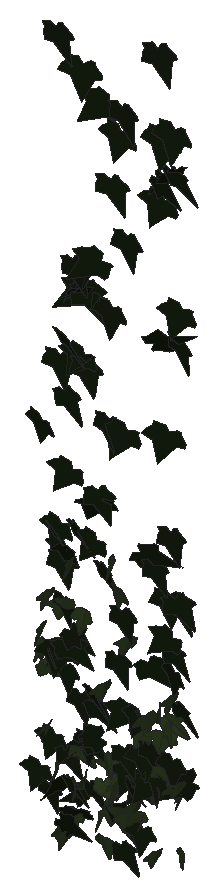
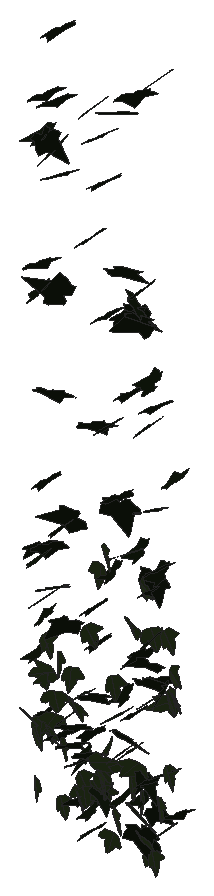
# SketchUp Ruby script. Lengths in inches.
U = 1.inch
M = Sketchup.active_model
def pt(a) = Geom::Point3d.new(a.map { |v| v * U })
def face(e, loops, mat)
  f = e.add_face(loops[0].map { |a| pt(a) })
  loops[1..].each { |l| e.add_face(l.map { |a| pt(a) }).erase! }
  f.material = f.back_material = mat if mat
  f
end
# faces: each face lists its corners as indices into pts; further lists are holes
def faces(e, pts, list, mat = nil) = list.each { |f| face(e, (f[0].is_a?(Array) ? f : [f]).map { |l| l.map { |i| pts[i] } }, mat) }
# xy, xz, yz: faces in a plane at the given z, y or x. An outline is a flat list of corners, or four numbers for a rectangle; further outlines are holes
def ring(l) = l.size == 4 ? [[l[0], l[1]], [l[2], l[1]], [l[2], l[3]], [l[0], l[3]]] : l.each_slice(2).to_a
def flat(e, list, mat, &to3) = list.each { |f| face(e, (f[0].is_a?(Array) ? f : [f]).map { |l| ring(l).map { |u, v| to3.(u, v) } }, mat) }
def xy(e, z, list, mat = nil) = flat(e, list, mat) { |x, y| [x, y, z] }
def xz(e, y, list, mat = nil) = flat(e, list, mat) { |x, z| [x, y, z] }
def yz(e, x, list, mat = nil) = flat(e, list, mat) { |y, z| [x, y, z] }
def lines(e, pts, list) = list.each { |a, b| e.add_line(pt(pts[a]), pt(pts[b])) }
# prism: a flat outline (further loops are holes) pulled along v
def prism(e, loops, v, mat = nil)
  f = face(e, loops, mat); d = Geom::Vector3d.new(v.map { |x| x * U })
  f.pushpull(f.normal.samedirection?(d) ? d.length : -d.length)
end
def box(e, o, s, mat = nil) = prism(e, [[o, [o[0] + s[0], o[1], o[2]], [o[0] + s[0], o[1] + s[1], o[2]], [o[0], o[1] + s[1], o[2]]]], [0, 0, s[2]], mat)
def at(x, y, z, deg = 0) = Geom::Transformation.translation(pt([x, y, z])) * Geom::Transformation.rotation(ORIGIN, Z_AXIS, deg.degrees)
def axes(o, x, y, z) = Geom::Transformation.new([*x, 0, *y, 0, *z, 0, *pt(o).to_a, 1])
def part(name) = M.definitions.add(name)
# library, detail: a bought-in or finely detailed component or shape, given as its bounding box
def library(name, o, s) = part(name).tap { |d| box(d.entities, o, s) }
def detail(e, o, s) = box(e.add_group.entities, o, s)
def put(e, d, t, mat = nil) = e.add_instance(d, t).tap { |i| i.material = mat if mat }
def group(e, t, mat = nil) = e.add_group.tap { |g| g.transformation = t; g.material = mat if mat }.entities
root = M.entities
M.materials.add("1026 AP 7946 SUNNY SIDE UP").color = [254, 231, 186]
M.materials.add("efeu1").color = [18, 25, 13]
M.materials.add("efeu2").color = [43, 57, 29]
c1 = part("ivyleaf_9")
p = [[1.54,2.16,1.25],[1.36,2.04,1.19],[-0.21,0.99,0.68],[-0.71,1.11,0.82],[-0.85,0.86,0.67],[-0.8,0.17,0.21],
  [-0.9,-0.01,0.1],[-0.67,-0.16,-0.02],[-0.08,-0.08,-0.05],[-0.03,-0.6,-0.4],[0.65,-0.88,-0.66],[0.83,-0.6,-0.49],
  [1.29,-0.42,-0.43],[1.8125,-0.07,-0.26],[1.21,0.44,0.15]]
faces(c1.entities,p,[[0,1,2,3,4,5,6,7,8,9,10,11,12,13,14]],"efeu1")
c2 = part("ivyleaf_10")
p = [[0,0.5,-0.03],[-0.0625,2.02,-0.43],[-0.19,2.01,-0.46],[-0.54,1.05,-0.29],[-0.52,0.625,-0.18],[-0.83,0.76,-0.28],
  [-1.16,0.64,-0.33],[-1.15,0.33,-0.24],[-0.77,-0.39,0.02],[-0.3,-0.51,0.16],[0.04,-0.48,0.23],[-0.02,2.01,-0.4375],
  [-0.06,2.01,-0.43],[0.04,-0.49,0.23],[0.67,-0.49,0.14],[1.38,0.36,-0.2],[1.375,0.51,-0.24],[0.81,0.65,-0.19],
  [0.62,0.59,-0.15],[0.6,1.09,-0.28],[0.5,1.23,-0.31]]
faces(c2.entities,p,[[0,1,2,3,4,5,6,7,8,9,10],[11,12,0,13,14,15,16,17,18,19,20]],"efeu2")
put(root,c1,axes([126.55,212.5,293.42],[-0.23595,-0.32373,0.07815],[-0.0196,-0.0797,-0.36738],[0.52312,-0.149,0.02148]),"1026 AP 7946 SUNNY SIDE UP")
put(root,c2,axes([126.6,212.58,298.9375],[0.33541,-0.32342,0.04435],[0.00742,-0.05056,-0.39867],[0.51336,0.21204,-0.02322]),"1026 AP 7946 SUNNY SIDE UP")
put(root,c1,axes([126.43,212.75,308.94],[-0.07996,-0.33132,0.24837],[0.06056,-0.24759,-0.34096],[0.6432,-0.01787,0.06298]),"1026 AP 7946 SUNNY SIDE UP")
put(root,c2,axes([126.68,212.49,299.83],[0.19146,-0.33124,0.17534],[0.08492,-0.16347,-0.36448],[0.58076,0.1331,-0.00451]),"1026 AP 7946 SUNNY SIDE UP")
put(root,c2,axes([126.76,212.63,298.82],[0.18874,-0.3655,0.00071],[-0.00202,-0.00333,-0.39634],[0.57473,0.12002,-0.00162]),"1026 AP 7946 SUNNY SIDE UP")
put(root,c2,axes([126.86,212.58,295.33],[0.04072,-0.37809,-0.0197],[-0.00933,0.01661,-0.39029],[0.59504,0.02613,-0.00477]),"1026 AP 7946 SUNNY SIDE UP")
put(root,c2,axes([127.04,212.45,301.48],[-0.00893,-0.38837,0.07664],[0.00467,-0.07665,-0.40057],[0.62242,-0.005,0.00411]),"1026 AP 7946 SUNNY SIDE UP")
put(root,c1,axes([126.87,212.68,292.64],[0.09245,-0.36281,0.01679],[0.01263,-0.01729,-0.37871],[0.57108,0.05912,0.00566]),"1026 AP 7946 SUNNY SIDE UP")
put(root,c1,axes([127.21,212.57,295.04],[-0.22827,-0.32169,0.12073],[0.01396,-0.13272,-0.35918],[0.53916,-0.13276,0.06041]),"1026 AP 7946 SUNNY SIDE UP")
put(root,c1,axes([127.27,212.25,299.08],[0.34526,-0.127,-0.30141],[-0.36637,0.17741,-0.25908],[0.34095,0.31924,0.02682]),"1026 AP 7946 SUNNY SIDE UP")
put(root,c2,axes([127.05,212.27,298.3125],[-0.29857,-0.12669,-0.31996],[0.46627,0.10165,-0.22943],[0.24425,-0.34891,0.04685]),"1026 AP 7946 SUNNY SIDE UP")
put(root,c2,axes([127.45,212.39,293.61],[0.10401,-0.31533,-0.20418],[-0.06261,0.19233,-0.33079],[0.58077,0.07721,0.00091]),"1026 AP 7946 SUNNY SIDE UP")
put(root,c1,axes([127.35,212.77,304.55],[-0.20686,-0.34979,0.14767],[-0.03951,-0.14544,-0.38493],[0.59429,-0.13143,0.02581]),"1026 AP 7946 SUNNY SIDE UP")
put(root,c1,axes([127.13,212.6,304.4],[0.4088,-0.31305,0.04436],[0.01422,-0.05066,-0.41871],[0.49707,0.25891,-0.0245]),"1026 AP 7946 SUNNY SIDE UP")
put(root,c1,axes([127.34,212.79,312.13],[-0.07721,-0.4209,-0.01707],[0.03892,0.01137,-0.43582],[0.66105,-0.04983,0.02367]),"1026 AP 7946 SUNNY SIDE UP")
put(root,c1,axes([127.73,212.45,293.22],[-0.14938,0.12869,-0.33624],[0.15491,-0.31553,-0.15919],[-0.53058,-0.12835,0.04819]),"1026 AP 7946 SUNNY SIDE UP")
put(root,c2,axes([127.68,212.5,291.06],[-0.0168,-0.36717,-0.02915],[0.02359,0.02577,-0.37798],[0.57833,-0.01172,0.01457]),"1026 AP 7946 SUNNY SIDE UP")
put(root,c1,axes([127.8,212.3,303.91],[0.42656,0.03098,-0.31665],[-0.45801,-0.11133,-0.27689],[-0.16267,0.3947,-0.05074]),"1026 AP 7946 SUNNY SIDE UP")
put(root,c1,axes([127.62,212.32,299.22],[-0.33432,-0.31974,-0.07946],[0.07534,0.05857,-0.39516],[0.511,-0.21783,0.00627]),"1026 AP 7946 SUNNY SIDE UP")
put(root,c1,axes([127.39,212.52,327.11],[0.15416,-0.46374,-0.03363],[0.00581,0.03145,-0.48801],[0.73069,0.09759,0.01097]),"1026 AP 7946 SUNNY SIDE UP")
put(root,c2,axes([127.81,212.42,301.33],[-0.34287,-0.31244,0.0685],[-0.01836,-0.0748,-0.3915],[0.50254,-0.2159,0.03244]),"1026 AP 7946 SUNNY SIDE UP")
put(root,c1,axes([127.97,212.71,299.18],[-0.54854,-0.15041,0.05138],[-0.05926,-0.04051,-0.39094],[0.24246,-0.35019,0.0207]),"1026 AP 7946 SUNNY SIDE UP")
put(root,c1,axes([127.82,212.875,307.15],[-0.38359,-0.29355,0.15153],[-0.00447,-0.18329,-0.37848],[0.51744,-0.21919,0.10907]),"1026 AP 7946 SUNNY SIDE UP")
put(root,c1,axes([127.58,212.71,301.23],[0.09658,-0.36927,0.11341],[0.01646,-0.11196,-0.38622],[0.60663,0.06183,-0.00757]),"1026 AP 7946 SUNNY SIDE UP")
put(root,c1,axes([127.48,212.75,313.14],[0.3575,-0.34872,0.11011],[0.08537,-0.09455,-0.42937],[0.56804,0.23368,-0.00477]),"1026 AP 7946 SUNNY SIDE UP")
put(root,c1,axes([127.75,212.43,303.33],[-0.03951,-0.39302,-0.05098],[0.01819,0.0466,-0.40534],[0.62217,-0.02632,0.00862]),"1026 AP 7946 SUNNY SIDE UP")
put(root,c1,axes([127.76,212.65,298.3],[-0.01319,-0.37307,0.08078],[0.00888,-0.08066,-0.38483],[0.60006,-0.00701,0.00747]),"1026 AP 7946 SUNNY SIDE UP")
put(root,c1,axes([128.1875,212.42,294.53],[-0.13272,0.35364,-0.04935],[0.00908,-0.04993,-0.37479],[-0.5615,-0.08439,0.0056]),"1026 AP 7946 SUNNY SIDE UP")
put(root,c2,axes([128.08,212.36,290.97],[-0.03457,-0.33319,0.12651],[-0.00755,-0.12465,-0.34471],[0.55935,-0.02228,0.00316]),"1026 AP 7946 SUNNY SIDE UP")
put(root,c1,axes([127.84,212.59,294.56],[0.11098,-0.3296,-0.16907],[-0.03247,0.16139,-0.34608],[0.57674,0.07251,0.01305]),"1026 AP 7946 SUNNY SIDE UP")
put(root,c1,axes([128.3,212.51,292.04],[0.27193,0.24171,-0.20631],[-0.22522,-0.14444,-0.30578],[-0.44075,0.22294,0.02896]),"1026 AP 7946 SUNNY SIDE UP")
put(root,c1,axes([127.94,212.37,310.88],[0.18142,-0.39495,-0.10808],[-0.01788,0.10354,-0.42289],[0.64142,0.1146,0.01878]),"1026 AP 7946 SUNNY SIDE UP")
put(root,c2,axes([128.24,212.42,303.34],[0.1718,-0.33223,0.20225],[0.07781,-0.19227,-0.36123],[0.60331,0.11941,-0.011]),"1026 AP 7946 SUNNY SIDE UP")
put(root,c2,axes([128.14,212.66,291.8],[0.51466,-0.13599,0.09309],[0.11502,-0.06077,-0.36442],[0.23028,0.33428,-0.02603]),"1026 AP 7946 SUNNY SIDE UP")
put(root,c1,axes([128.37,212.9375,312.52],[-0.36904,-0.30707,0.17452],[0.01169,-0.21008,-0.37902],[0.55266,-0.20061,0.12455]),"1026 AP 7946 SUNNY SIDE UP")
put(root,c1,axes([127.98,212.19,291.61],[0.15793,-0.05832,-0.36928],[0.54199,0.13141,0.07831],[0.17822,-0.34796,0.08909]),"1026 AP 7946 SUNNY SIDE UP")
put(root,c1,axes([128.79,212.53,292.96],[-0.45379,0.21622,0.02136],[-0.0486,-0.0088,-0.37062],[-0.33789,-0.28912,0.02462]),"1026 AP 7946 SUNNY SIDE UP")
put(root,c1,axes([128.83,212.64,315.69],[-0.63747,-0.12167,0.11294],[-0.14473,-0.07503,-0.43414],[0.21389,-0.4134,0.04285]),"1026 AP 7946 SUNNY SIDE UP")
put(root,c1,axes([128.24,212.21,293.53],[0.35945,-0.28335,-0.02805],[-0.00497,0.03033,-0.37449],[0.44733,0.22802,0.01838]),"1026 AP 7946 SUNNY SIDE UP")
put(root,c1,axes([128.33,212.29,300.24],[0.17276,-0.24167,-0.29422],[-0.05301,0.28865,-0.26458],[0.58423,0.09766,0.06299]),"1026 AP 7946 SUNNY SIDE UP")
put(root,c2,axes([128.6,212.1,293.4375],[0.24088,-0.2995,-0.1755],[0.00508,0.18589,-0.33597],[0.54044,0.13174,0.08138]),"1026 AP 7946 SUNNY SIDE UP")
put(root,c1,axes([128.2,212.2,299.72],[-0.00632,-0.25513,-0.30523],[0.38811,0.22659,-0.20413],[0.4746,-0.18869,0.16287]),"1026 AP 7946 SUNNY SIDE UP")
put(root,c1,axes([128.36,212.33,316.98],[0.16521,-0.42567,-0.08107],[-0.04085,0.07214,-0.45119],[0.67876,0.10795,-0.00742]),"1026 AP 7946 SUNNY SIDE UP")
put(root,c1,axes([128.34,212.2,315.5],[0.44614,0.20815,0.29101],[0.35913,0.16422,-0.36156],[-0.41688,0.36423,-0.00004]),"1026 AP 7946 SUNNY SIDE UP")
put(root,c1,axes([128.34,212.4375,304.98],[0.39163,-0.32856,0.02118],[-0.00849,-0.03219,-0.42422],[0.51775,0.24799,-0.02298]),"1026 AP 7946 SUNNY SIDE UP")
put(root,c1,axes([128.82,212.5,316.43],[-0.50429,0.16828,-0.25375],[0.28854,-0.1756,-0.36932],[-0.3714,-0.36492,0.05762]),"1026 AP 7946 SUNNY SIDE UP")
put(root,c2,axes([128.64,212.5,294.9375],[-0.46994,-0.11756,-0.1857],[0.31136,-0.03218,-0.31797],[0.13027,-0.34719,0.09007]),"1026 AP 7946 SUNNY SIDE UP")
put(root,c1,axes([128.65,212.47,297.38],[-0.01118,-0.38399,0.00314],[0.01125,-0.00536,-0.39561],[0.60374,-0.00701,0.00743]),"1026 AP 7946 SUNNY SIDE UP")
put(root,c1,axes([128.72,212.5,325.93],[-0.26005,-0.43802,-0.06153],[0.03681,0.05235,-0.48202],[0.69362,-0.167,0.00251]),"1026 AP 7946 SUNNY SIDE UP")
put(root,c1,axes([128.68,212.73,312.28],[-0.0145,-0.4248,-0.05453],[0.02532,0.05015,-0.43717],[0.67219,-0.01105,0.01529]),"1026 AP 7946 SUNNY SIDE UP")
put(root,c2,axes([128.89,212.3,301.22],[0.52051,-0.17099,0.11087],[0.12009,-0.08732,-0.38203],[0.29499,0.33726,-0.04009]),"1026 AP 7946 SUNNY SIDE UP")
put(root,c2,axes([129.09,212.11,293.97],[0.06079,-0.3589,-0.16106],[-0.01703,0.15401,-0.37094],[0.61405,0.0398,0.00566]),"1026 AP 7946 SUNNY SIDE UP")
put(root,c1,axes([128.83,212.58,315.85],[0.04497,-0.40932,-0.23623],[0.01133,0.22777,-0.42086],[0.73587,0.0215,0.02092]),"1026 AP 7946 SUNNY SIDE UP")
put(root,c1,axes([128.91,212.53,295.48],[-0.01156,-0.3561,0.11719],[0.01252,-0.11592,-0.36747],[0.58865,-0.00453,0.01012]),"1026 AP 7946 SUNNY SIDE UP")
put(root,c1,axes([129.21,212.66,304.52],[-0.31576,-0.29214,0.19796],[-0.02821,-0.2145,-0.35349],[0.55054,-0.17854,0.09542]),"1026 AP 7946 SUNNY SIDE UP")
put(root,c1,axes([129.71,212.25,295.93],[-0.55749,0.08912,0.09035],[-0.14611,-0.01363,-0.37497],[-0.13071,-0.36485,0.03381]),"1026 AP 7946 SUNNY SIDE UP")
put(root,c1,axes([129.09,212.49,295.52],[0.24991,-0.29403,-0.17339],[-0.05376,0.16921,-0.34019],[0.52869,0.15619,0.04737]),"1026 AP 7946 SUNNY SIDE UP")
put(root,c1,axes([129.07,212.61,293.37],[0.25653,-0.33574,-0.01823],[0.0131,0.02158,-0.38403],[0.52834,0.16248,0.01838]),"1026 AP 7946 SUNNY SIDE UP")
put(root,c1,axes([129.64,212.39,317.4375],[-0.61147,-0.17293,0.12486],[-0.15089,-0.08382,-0.43735],[0.29678,-0.39891,0.03489]),"1026 AP 7946 SUNNY SIDE UP")
put(root,c1,axes([129.58,212.27,306.59],[0.28992,0.29142,-0.24465],[-0.19454,-0.20468,-0.35644],[-0.55993,0.22201,-0.00284]),"1026 AP 7946 SUNNY SIDE UP")
put(root,c1,axes([129.24,212.26,297.92],[0.3652,-0.30263,0.02631],[-0.00594,-0.03718,-0.39234],[0.47775,0.23087,-0.02499]),"1026 AP 7946 SUNNY SIDE UP")
put(root,c1,axes([129.26,212.55,297.16],[0.24746,-0.32151,-0.1333],[0.02866,0.14766,-0.35937],[0.54313,0.13869,0.07969]),"1026 AP 7946 SUNNY SIDE UP")
put(root,c2,axes([129.67,212.47,292.23],[0.20428,-0.34844,-0.04114],[-0.02144,0.03542,-0.38289],[0.55071,0.13063,0.00035]),"1026 AP 7946 SUNNY SIDE UP")
put(root,c1,axes([129.93,212.52,324.67],[-0.57682,-0.23976,0.16564],[-0.05355,-0.22421,-0.42221],[0.45196,-0.33256,0.16139]),"1026 AP 7946 SUNNY SIDE UP")
put(root,c1,axes([129.625,212.33,306.99],[0.00902,-0.3858,-0.15729],[0.00518,0.15054,-0.39658],[0.65113,0.00415,0.00533]),"1026 AP 7946 SUNNY SIDE UP")
put(root,c2,axes([129.9,212.33,298.31],[-0.11201,-0.38349,-0.02884],[0.01885,0.02403,-0.40162],[0.60407,-0.07186,0.00718]),"1026 AP 7946 SUNNY SIDE UP")
put(root,c2,axes([129.87,212.49,291.23],[-0.52752,0.13791,-0.02505],[0.01487,-0.04268,-0.3721],[-0.21991,-0.3337,0.03492]),"1026 AP 7946 SUNNY SIDE UP")
put(root,c1,axes([129.7,212.49,303.55],[0.32732,-0.34261,0.02159],[-0.00756,-0.02969,-0.41268],[0.53987,0.20731,-0.01887]),"1026 AP 7946 SUNNY SIDE UP")
put(root,c2,axes([130.44,212.73,294.56],[0.10562,0.12642,0.35521],[-0.40813,-0.23062,0.13814],[0.40703,-0.26405,0.04634]),"1026 AP 7946 SUNNY SIDE UP")
put(root,c1,axes([129.95,212.59,310.22],[0.00581,-0.41861,0.02893],[0.00323,-0.03044,-0.43144],[0.65996,0.00384,0.00186]),"1026 AP 7946 SUNNY SIDE UP")
put(root,c1,axes([130.07,212.65,315.3],[-0.1213,-0.41393,0.09497],[-0.00942,-0.09502,-0.43417],[0.66756,-0.07655,0.01113]),"1026 AP 7946 SUNNY SIDE UP")
put(root,c1,axes([130.49,212.35,292.85],[0.02227,0.31872,0.18351],[-0.13176,0.17457,-0.31713],[-0.55737,-0.02853,0.0823]),"1026 AP 7946 SUNNY SIDE UP")
put(root,c2,axes([130.26,212.11,295.22],[-0.12069,0.35931,-0.03595],[0.0033,-0.03731,-0.37868],[-0.56794,-0.07657,0.00544]),"1026 AP 7946 SUNNY SIDE UP")
put(root,c2,axes([130.41,212.4375,293.625],[0.21895,-0.33461,-0.07604],[-0.01643,0.07345,-0.37246],[0.5379,0.13844,0.01958]),"1026 AP 7946 SUNNY SIDE UP")
put(root,c2,axes([130.42,212.2,304.1],[0.24568,-0.36509,-0.05365],[-0.00747,0.05231,-0.40847],[0.57938,0.15549,0.01749]),"1026 AP 7946 SUNNY SIDE UP")
put(root,c2,axes([130.28,211.94,293.88],[0.33987,0.20659,-0.24315],[0.2377,0.18416,0.30823],[0.43373,-0.2628,0.02161]),"1026 AP 7946 SUNNY SIDE UP")
put(root,c2,axes([130.5625,212.42,293.75],[-0.04545,-0.2433,0.29485],[0.01739,-0.28885,-0.2523],[0.59206,-0.01019,0.03004]),"1026 AP 7946 SUNNY SIDE UP")
put(root,c2,axes([130.62,212.21,292.97],[-0.32381,-0.2959,0.05889],[-0.02953,-0.05854,-0.37128],[0.47346,-0.20602,0.01712]),"1026 AP 7946 SUNNY SIDE UP")
put(root,c1,axes([130.29,212.32,321.3125],[0.04878,-0.44374,-0.07678],[0.06641,0.07474,-0.45528],[0.70374,0.0237,0.04829]),"1026 AP 7946 SUNNY SIDE UP")
put(root,c2,axes([130.54,212.34,293.99],[0.1522,-0.27008,0.24506],[0.13226,-0.22417,-0.29686],[0.55188,0.1282,0.00356]),"1026 AP 7946 SUNNY SIDE UP")
put(root,c1,axes([130.49,212.6875,323.41],[-0.20937,-0.4136,0.15418],[0.0078,-0.1602,-0.44549],[0.69283,-0.12318,0.05161]),"1026 AP 7946 SUNNY SIDE UP")
put(root,c1,axes([130.38,212.16,292.95],[0.36519,-0.28335,-0.05435],[-0.03676,0.04694,-0.37697],[0.45125,0.23313,0.01327]),"1026 AP 7946 SUNNY SIDE UP")
put(root,c2,axes([130.84,212.0625,303.08],[-0.51613,0.2193,0.07821],[-0.14105,-0.00092,-0.40344],[-0.33585,-0.33663,0.04925]),"1026 AP 7946 SUNNY SIDE UP")
put(root,c1,axes([130.79,212.61,310.02],[-0.46525,-0.30722,0.01768],[0.01843,-0.03745,-0.4382],[0.48363,-0.29412,0.0337]),"1026 AP 7946 SUNNY SIDE UP")
put(root,c1,axes([130.89,212.62,297.42],[-0.45732,-0.22849,0.07472],[-0.04561,-0.08168,-0.37862],[0.37479,-0.28873,0.0451]),"1026 AP 7946 SUNNY SIDE UP")
put(root,c1,axes([130.57,212.69,301.71],[0.054,-0.39502,-0.03342],[-0.00488,0.03005,-0.40831],[0.62292,0.03448,-0.0003]),"1026 AP 7946 SUNNY SIDE UP")
put(root,c2,axes([130.86,212.74,300.51],[-0.13601,-0.36046,0.13026],[-0.00001,-0.13173,-0.38148],[0.60172,-0.08148,0.02944]),"1026 AP 7946 SUNNY SIDE UP")
put(root,c1,axes([130.67,212.26,299.89],[0.06804,-0.3887,-0.07295],[-0.02539,0.06722,-0.40242],[0.62012,0.0454,-0.00847]),"1026 AP 7946 SUNNY SIDE UP")
put(root,c1,axes([130.63,212.63,292.3],[0.32811,-0.30098,-0.04103],[-0.04664,0.02581,-0.37701],[0.47475,0.21055,-0.00868]),"1026 AP 7946 SUNNY SIDE UP")
put(root,c1,axes([130.76,212.72,318.71],[0.03033,-0.44582,0.02606],[-0.00002,-0.02785,-0.45987],[0.70237,0.01925,-0.00114]),"1026 AP 7946 SUNNY SIDE UP")
put(root,c1,axes([130.73,212.49,324.66],[0.13149,-0.45874,0.00221],[-0.00752,-0.0057,-0.48038],[0.72133,0.08357,-0.00541]),"1026 AP 7946 SUNNY SIDE UP")
put(root,c1,axes([130.76,212.45,291.26],[0.15403,-0.33363,-0.13048],[0.00397,0.13004,-0.35544],[0.56006,0.09083,0.03841]),"1026 AP 7946 SUNNY SIDE UP")
put(root,c1,axes([131.04,212.6875,294.71],[-0.37693,-0.28333,0.02178],[0.02688,-0.04408,-0.3802],[0.44613,-0.23672,0.04131]),"1026 AP 7946 SUNNY SIDE UP")
put(root,c1,axes([130.89,212.43,295.71],[-0.00046,-0.35047,-0.13261],[-0.00134,0.12673,-0.36031],[0.586,0.00002,-0.00093]),"1026 AP 7946 SUNNY SIDE UP")
put(root,c2,axes([131.26,212.53,292.89],[-0.47423,-0.21614,0.04423],[0.00452,-0.07864,-0.37678],[0.34685,-0.2945,0.06538]),"1026 AP 7946 SUNNY SIDE UP")
put(root,c2,axes([131.28,212.17,292.93],[-0.30738,-0.3137,0.02305],[0.00773,-0.03148,-0.38036],[0.49466,-0.19444,0.02027]),"1026 AP 7946 SUNNY SIDE UP")
put(root,c2,axes([131.45,212.4,293.39],[-0.04725,-0.36663,0.08242],[0.0051,-0.0826,-0.37931],[0.59073,-0.02861,0.00987]),"1026 AP 7946 SUNNY SIDE UP")
put(root,c1,axes([131.35,212.78,297.27],[-0.17949,-0.31079,0.1898],[0.00206,-0.19537,-0.33662],[0.56951,-0.09724,0.06104]),"1026 AP 7946 SUNNY SIDE UP")
put(root,c1,axes([131.33,212.16,294.44],[0.40808,-0.17349,-0.22856],[-0.26834,0.14145,-0.3202],[0.35076,0.31005,0.02095]),"1026 AP 7946 SUNNY SIDE UP")
put(root,c2,axes([131.56,212.58,292.73],[0.2675,-0.33436,-0.03632],[-0.02288,0.03003,-0.3863],[0.52787,0.17074,0.00166]),"1026 AP 7946 SUNNY SIDE UP")
put(root,c1,axes([131.56,212.76,294.13],[-0.29599,-0.25224,0.18526],[-0.06961,-0.188,-0.31798],[0.48342,-0.18151,0.06764]),"1026 AP 7946 SUNNY SIDE UP")
put(root,c2,axes([131.63,212.63,296.77],[0.53428,-0.17371,-0.00435],[-0.028,-0.02774,-0.39184],[0.27176,0.33866,-0.03181]),"1026 AP 7946 SUNNY SIDE UP")
put(root,c1,axes([131.66,212.57,292.34],[-0.16443,-0.3512,0.01721],[0.00529,-0.02051,-0.37751],[0.55298,-0.10424,0.00873]),"1026 AP 7946 SUNNY SIDE UP")
put(root,c1,axes([131.76,212.67,295.75],[-0.27686,-0.3307,-0.07247],[0.15083,0.02506,-0.37868],[0.50914,-0.18725,0.07278]),"1026 AP 7946 SUNNY SIDE UP")
put(root,c1,axes([132.16,212.51,294.64],[-0.38855,-0.26782,0.11638],[-0.04166,-0.12886,-0.37017],[0.45609,-0.23993,0.06534]),"1026 AP 7946 SUNNY SIDE UP")
put(root,c1,axes([131.9375,212.64,296.15],[0.12078,-0.37331,-0.03756],[-0.01944,0.03251,-0.3924],[0.58915,0.0776,-0.00525]),"1026 AP 7946 SUNNY SIDE UP")
put(root,c2,axes([132.25,212.1,297.81],[-0.17117,-0.36797,-0.11422],[0.08769,0.0967,-0.39391],[0.59694,-0.11972,0.02511]),"1026 AP 7946 SUNNY SIDE UP")
put(root,c1,axes([131.94,212.23,305.11],[0.20862,-0.00081,-0.39424],[0.31583,0.34491,0.07301],[0.51219,-0.21235,0.11556]),"1026 AP 7946 SUNNY SIDE UP")
put(root,c1,axes([132.29,212.27,300.2],[-0.02037,-0.20157,-0.35652],[0.07096,0.34216,-0.20574],[0.62417,-0.04548,0.01176]),"1026 AP 7946 SUNNY SIDE UP")
put(root,c1,axes([132.52,212.81,320.98],[-0.33531,-0.3653,0.15756],[0.00362,-0.17712,-0.42776],[0.62396,-0.19528,0.08715]),"1026 AP 7946 SUNNY SIDE UP")
put(root,c2,axes([132.64,212.69,296.86],[-0.48974,-0.20313,0.07747],[0.00712,-0.13961,-0.36444],[0.34115,-0.2887,0.11881]),"1026 AP 7946 SUNNY SIDE UP")
put(root,c2,axes([132.65,212.1875,291.76],[-0.07166,-0.35748,0.00638],[0.00331,-0.00855,-0.37129],[0.56224,-0.04551,0.003]),"1026 AP 7946 SUNNY SIDE UP")
put(root,c1,axes([132.375,212.7,327.81],[0.02978,-0.46148,-0.10639],[-0.00376,0.10063,-0.47523],[0.74269,0.01901,0.00186]),"1026 AP 7946 SUNNY SIDE UP")
put(root,c2,axes([132.69,212.16,294.54],[0.34319,-0.26658,-0.15165],[-0.08383,0.143,-0.351],[0.47028,0.22003,0.0481]),"1026 AP 7946 SUNNY SIDE UP")
put(root,c1,axes([132.41,212.38,304.65],[0.11651,-0.39389,-0.08587],[-0.01849,0.08033,-0.41242],[0.63208,0.07496,0.00376]),"1026 AP 7946 SUNNY SIDE UP")
put(root,c1,axes([132.59,212.6,295.01],[-0.2047,-0.35135,0.03494],[-0.00046,-0.03817,-0.386],[0.55534,-0.12954,0.01256]),"1026 AP 7946 SUNNY SIDE UP")
put(root,c2,axes([132.84,212.12,298.3],[0.12546,-0.34604,-0.17608],[0.03187,0.17607,-0.36063],[0.60467,0.06252,0.05554]),"1026 AP 7946 SUNNY SIDE UP")
put(root,c1,axes([132.64,212.35,322.19],[0.37455,-0.31859,-0.23362],[-0.1742,0.19747,-0.40779],[0.58799,0.26145,0.028]),"1026 AP 7946 SUNNY SIDE UP")
put(root,c1,axes([133.15,212.71,322.5625],[-0.20105,0.28835,-0.34018],[0.11454,-0.32693,-0.32347],[-0.68171,-0.13997,0.04597]),"1026 AP 7946 SUNNY SIDE UP")
put(root,c1,axes([132.86,212.45,324.1875],[-0.2173,-0.44285,0.04317],[0.01219,-0.0489,-0.47767],[0.69972,-0.13668,0.02173]),"1026 AP 7946 SUNNY SIDE UP")
put(root,c1,axes([132.99,212.55,310.75],[-0.49238,-0.2793,-0.09276],[0.17619,0.00545,-0.42635],[0.42564,-0.32535,0.06918]),"1026 AP 7946 SUNNY SIDE UP")
put(root,c1,axes([133.16,212.51,301.55],[-0.41757,-0.22272,0.19156],[-0.08595,-0.21077,-0.33942],[0.44935,-0.24728,0.11309]),"1026 AP 7946 SUNNY SIDE UP")
put(root,c2,axes([132.97,212.66,295.22],[0.47522,-0.21334,0.07181],[0.08245,-0.04865,-0.38127],[0.34375,0.3066,-0.00782]),"1026 AP 7946 SUNNY SIDE UP")
put(root,c2,axes([132.93,212.39,295.6],[-0.3737,-0.24124,-0.16776],[0.26667,0.05399,-0.33993],[0.37046,-0.28221,0.07546]),"1026 AP 7946 SUNNY SIDE UP")
put(root,c2,axes([133.2,212.48,297.52],[0.12541,0.36539,-0.06134],[-0.05281,-0.05564,-0.38503],[-0.58026,0.08403,0.02179]),"1026 AP 7946 SUNNY SIDE UP")
put(root,c1,axes([133.18,212.42,303.49],[-0.22359,-0.36745,-0.10864],[0.05696,0.09682,-0.40533],[0.5975,-0.14674,-0.00201]),"1026 AP 7946 SUNNY SIDE UP")
put(root,c1,axes([133.18,212.58,295.9375],[-0.07564,-0.37761,0.03637],[-0.01131,-0.03683,-0.39236],[0.59656,-0.04858,-0.00283]),"1026 AP 7946 SUNNY SIDE UP")
put(root,c1,axes([132.85,211.96,315.01],[0.15847,-0.04229,0.44392],[0.66986,0.09011,-0.09296],[-0.12378,0.43351,0.0653]),"1026 AP 7946 SUNNY SIDE UP")
put(root,c1,axes([133.22,212.64,324.45],[-0.18621,-0.44723,0.04564],[0.00803,-0.04977,-0.47656],[0.70703,-0.11722,0.01743]),"1026 AP 7946 SUNNY SIDE UP")
put(root,c2,axes([133.42,212.29,299],[0.00222,-0.39003,0.06075],[0.01198,-0.06115,-0.4021],[0.62067,0.00257,0.00754]),"1026 AP 7946 SUNNY SIDE UP")
put(root,c2,axes([133.04,212.53,297.74],[0.31718,0.05337,0.3256],[0.47204,0.0984,-0.21413],[-0.1753,0.36154,0.01253]),"1026 AP 7946 SUNNY SIDE UP")
put(root,c1,axes([133.34,212.28,306.4375],[0.04417,-0.41047,-0.06969],[-0.03455,0.0639,-0.4231],[0.65263,0.03117,-0.01768]),"1026 AP 7946 SUNNY SIDE UP")
put(root,c1,axes([133.28,212.41,301.08],[0.20511,-0.36409,-0.10652],[-0.00216,0.10674,-0.3963],[0.59425,0.12605,0.03533]),"1026 AP 7946 SUNNY SIDE UP")
put(root,c1,axes([133.37,212.43,300.09],[0.00136,-0.31377,0.24508],[0.01366,-0.23961,-0.32458],[0.6207,0.00596,0.00661]),"1026 AP 7946 SUNNY SIDE UP")
put(root,c1,axes([133.21,212.58,322.59],[0.36289,-0.39634,-0.01696],[0.06151,0.03912,-0.46904],[0.62057,0.22789,0.05641]),"1026 AP 7946 SUNNY SIDE UP")
put(root,c1,axes([133.34,212.74,303.01],[0.18839,-0.38188,0.00147],[0.00679,-0.00241,-0.41232],[0.60046,0.11984,0.00421]),"1026 AP 7946 SUNNY SIDE UP")
put(root,c1,axes([133.6,212.59,316.47],[-0.2876,-0.38588,0.08718],[-0.02071,-0.08965,-0.43964],[0.62158,-0.18153,0.02569]),"1026 AP 7946 SUNNY SIDE UP")
put(root,c2,axes([133.74,212.17,295.15],[-0.22689,-0.33996,-0.07172],[0.04683,0.06089,-0.38009],[0.54303,-0.14729,0.00281]),"1026 AP 7946 SUNNY SIDE UP")
put(root,c2,axes([133.74,212.52,294.71],[0.14056,-0.36215,0.03156],[-0.00006,-0.03367,-0.38439],[0.57176,0.08903,-0.0078]),"1026 AP 7946 SUNNY SIDE UP")
put(root,c1,axes([133.53,212.42,303.42],[0.02579,-0.34491,-0.22536],[0.06289,0.21728,-0.35174],[0.63748,-0.00748,0.04382]),"1026 AP 7946 SUNNY SIDE UP")
put(root,c1,axes([134.16,212.51,295.33],[-0.66505,0.18973,-0.05659],[0.05276,-0.06149,-0.47594],[-0.30655,-0.42219,0.04086]),"1026 AP 7946 SUNNY SIDE UP")
put(root,c1,axes([133.49,212.5625,298.53],[0.31334,-0.33746,-0.00661],[0.01903,0.01237,-0.4033],[0.53033,0.19894,0.01838]),"1026 AP 7946 SUNNY SIDE UP")
put(root,c1,axes([133.57,212.48,315.1],[0.16373,-0.40703,0.10649],[0.02161,-0.10552,-0.43325],[0.66088,0.10429,-0.01221]),"1026 AP 7946 SUNNY SIDE UP")
put(root,c2,axes([134,212.16,292.14],[0.31665,-0.2727,-0.13211],[0.00606,0.1548,-0.33606],[0.47276,0.18066,0.09279]),"1026 AP 7946 SUNNY SIDE UP")
